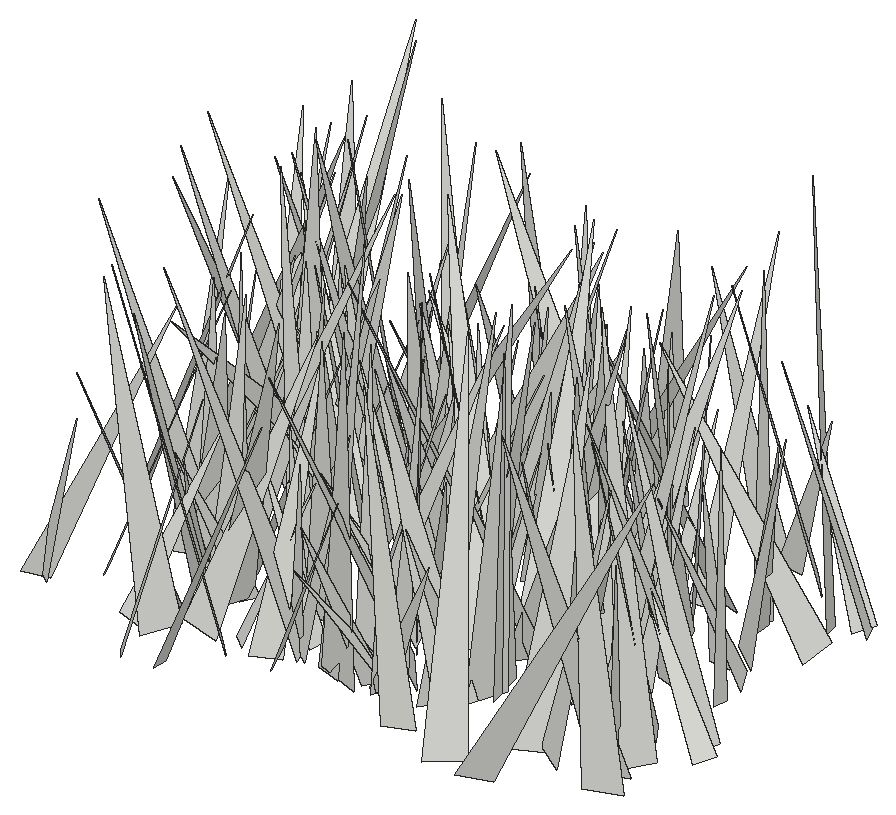
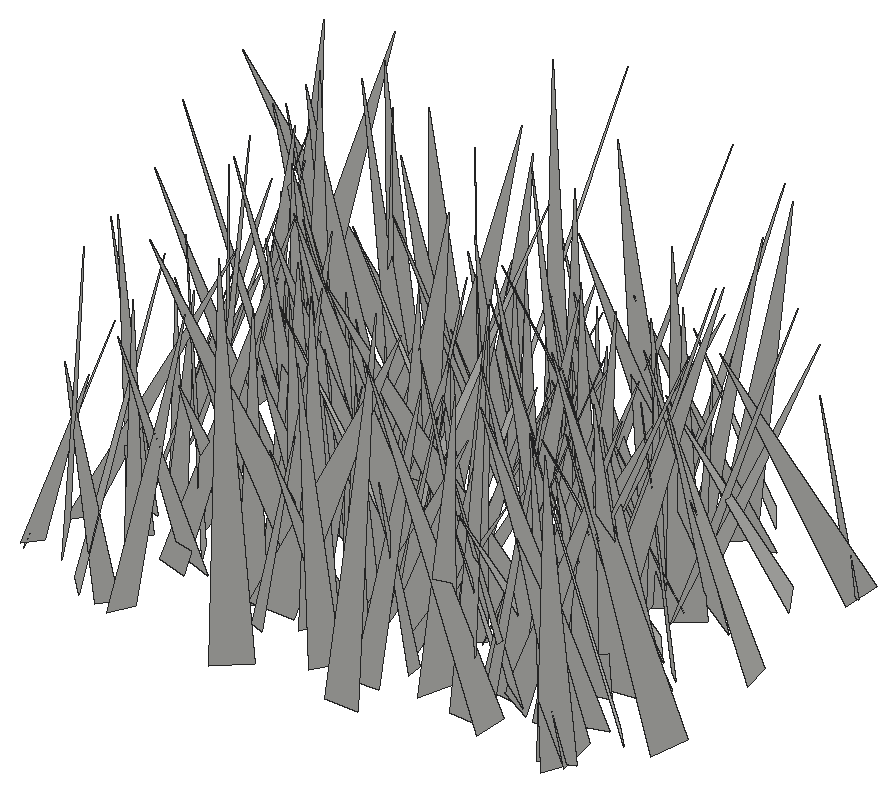
# SketchUp Ruby script. Lengths in inches.
U = 1.inch
M = Sketchup.active_model
def pt(a) = Geom::Point3d.new(a.map { |v| v * U })
def face(e, loops, mat)
  f = e.add_face(loops[0].map { |a| pt(a) })
  loops[1..].each { |l| e.add_face(l.map { |a| pt(a) }).erase! }
  f.material = f.back_material = mat if mat
  f
end
# faces: each face lists its corners as indices into pts; further lists are holes
def faces(e, pts, list, mat = nil) = list.each { |f| face(e, (f[0].is_a?(Array) ? f : [f]).map { |l| l.map { |i| pts[i] } }, mat) }
# xy, xz, yz: faces in a plane at the given z, y or x. An outline is a flat list of corners, or four numbers for a rectangle; further outlines are holes
def ring(l) = l.size == 4 ? [[l[0], l[1]], [l[2], l[1]], [l[2], l[3]], [l[0], l[3]]] : l.each_slice(2).to_a
def flat(e, list, mat, &to3) = list.each { |f| face(e, (f[0].is_a?(Array) ? f : [f]).map { |l| ring(l).map { |u, v| to3.(u, v) } }, mat) }
def xy(e, z, list, mat = nil) = flat(e, list, mat) { |x, y| [x, y, z] }
def xz(e, y, list, mat = nil) = flat(e, list, mat) { |x, z| [x, y, z] }
def yz(e, x, list, mat = nil) = flat(e, list, mat) { |y, z| [x, y, z] }
def lines(e, pts, list) = list.each { |a, b| e.add_line(pt(pts[a]), pt(pts[b])) }
# prism: a flat outline (further loops are holes) pulled along v
def prism(e, loops, v, mat = nil)
  f = face(e, loops, mat); d = Geom::Vector3d.new(v.map { |x| x * U })
  f.pushpull(f.normal.samedirection?(d) ? d.length : -d.length)
end
def box(e, o, s, mat = nil) = prism(e, [[o, [o[0] + s[0], o[1], o[2]], [o[0] + s[0], o[1] + s[1], o[2]], [o[0], o[1] + s[1], o[2]]]], [0, 0, s[2]], mat)
def at(x, y, z, deg = 0) = Geom::Transformation.translation(pt([x, y, z])) * Geom::Transformation.rotation(ORIGIN, Z_AXIS, deg.degrees)
def axes(o, x, y, z) = Geom::Transformation.new([*x, 0, *y, 0, *z, 0, *pt(o).to_a, 1])
def part(name) = M.definitions.add(name)
# library, detail: a bought-in or finely detailed component or shape, given as its bounding box
def library(name, o, s) = part(name).tap { |d| box(d.entities, o, s) }
def detail(e, o, s) = box(e.add_group.entities, o, s)
def put(e, d, t, mat = nil) = e.add_instance(d, t).tap { |i| i.material = mat if mat }
def group(e, t, mat = nil) = e.add_group.tap { |g| g.transformation = t; g.material = mat if mat }.entities
root = M.entities
c1 = part("fur_instance\#9")
p = [[0.8125,0,1.79],[0.67,-0.02,1.48],[0,-0.11,0],[0,0.11,0]]
faces(c1.entities,p,[[0,1,2,3]])
put(root,c1,axes([93.47,217.7,-27.1],[-5.98098,3.27291,2.42019],[3.72115,6.13978,0.89298],[1.64993,-1.98304,6.75918]))
put(root,c1,axes([94.98,215.74,-27.1],[4.77629,1.47467,0.59608],[1.29577,-4.70156,1.24867],[-0.92247,1.03128,4.84029]))
put(root,c1,axes([93.41,215.47,-27.1],[3.76197,3.17485,0.58422],[2.97684,-3.75885,1.25811],[-1.24876,0.60394,4.75913]))
put(root,c1,axes([102.43,220.92,-27.1],[-6.0329,-5.73941,0.68236],[-5.34499,5.91535,2.49841],[2.19943,-1.36753,7.94322]))
put(root,c1,axes([97.98,218.64,-27.1],[5.19096,1.17327,0.15724],[1.14991,-4.82989,-1.92283],[0.28108,-1.90867,4.96239]))
put(root,c1,axes([95.97,218.12,-27.1],[-5.67662,-5.13617,1.32256],[-5.29359,5.60645,-0.94818],[0.32758,1.59402,7.59639]))
put(root,c1,axes([108.84,216.25,-27.1],[6.56364,-3.25708,1.01889],[-3.38805,-5.95385,2.79299],[0.40967,2.94467,6.77415]))
put(root,c1,axes([100.55,218.85,-27.1],[-1.23371,-7.71978,2.49826],[-7.92295,1.69122,1.31342],[1.75022,2.21429,7.70662]))
put(root,c1,axes([104.48,217.4,-27.1],[-1.23354,6.12021,2.2306],[6.48252,0.93032,1.03231],[-0.63996,-2.37312,6.15735]))
put(root,c1,axes([102.16,219.85,-27.1],[-3.24466,-1.65637,0.06319],[-1.44148,2.88818,1.68993],[0.81834,-1.47993,3.2273]))
put(root,c1,axes([101.77,219.4,-27.1],[1.92833,-3.54748,0.58332],[-3.33012,-2.01195,-1.22706],[-1.35468,-0.10385,3.84674]))
put(root,c1,axes([112.54,219.42,-27.1],[0.14854,-7.36709,1.66817],[-7.40985,-0.46607,-1.39849],[-1.46661,1.60862,7.23466]))
put(root,c1,axes([87.66,218.23,-27.1],[2.1321,2.91958,1.28602],[3.18698,-1.87905,-1.01782],[0.14466,-1.63367,3.46899]))
put(root,c1,axes([102.47,218.9,-27.1],[1.15805,-3.96128,0.43832],[-3.70743,-0.90324,1.63219],[1.46246,0.84697,3.79062]))
put(root,c1,axes([113.02,218.3,-27.1],[1.15068,-6.84996,3.27998],[-7.48842,-1.57649,-0.66528],[-1.26644,3.09791,6.914]))
put(root,c1,axes([98.26,219.91,-27.1],[-7.76303,-2.55675,1.09489],[-2.43873,7.81802,0.96517],[1.33728,-0.58482,8.11604]))
put(root,c1,axes([93.29,219.18,-27.1],[-3.10953,-4.00727,0.37973],[-3.98696,3.00024,-0.98706],[-0.55366,0.90108,4.97525]))
put(root,c1,axes([102.33,219.09,-27.1],[3.31226,-1.52366,0.97308],[-1.49474,-3.45052,-0.31491],[-1.01694,0.10903,3.63228]))
put(root,c1,axes([107.26,216.53,-27.1],[5.53383,-2.65462,5.00816],[-4.23304,-6.59023,1.18414],[-3.76962,3.5034,6.0223]))
put(root,c1,axes([92.13,217.6,-27.1],[0.26684,4.21608,0.5662],[4.07293,-0.08948,-1.25314],[1.22767,-0.6195,4.03438]))
put(root,c1,axes([105.17,219.86,-27.1],[4.68158,-4.31782,3.21331],[-4.18207,-5.59908,-1.43065],[-3.3881,0.94493,6.20597]))
put(root,c1,axes([104.95,220.79,-27.1],[4.08531,-1.79648,1.28746],[-1.24322,-4.1049,-1.78292],[-1.82737,-1.22355,4.09124]))
put(root,c1,axes([93.17,220.53,-27.1],[-2.27159,-6.08211,1.19958],[-6.16809,2.34544,0.21162],[0.62109,1.04786,6.48903]))
put(root,c1,axes([110.01,219.02,-27.1],[3.01267,4.99828,1.819],[5.31773,-2.78497,-1.15474],[0.11548,-2.15148,5.72063]))
put(root,c1,axes([94.23,220.75,-27.1],[7.12513,-3.29011,0.44393],[-3.26274,-7.13377,-0.50321],[-0.6135,-0.27186,7.83192]))
put(root,c1,axes([98,219.7,-27.1],[-1.12295,-3.74744,1.45837],[-3.89173,1.39395,0.58526],[1.01223,1.20198,3.86805]))
put(root,c1,axes([94.55,218.55,-27.1],[0.24671,6.36494,1.6516],[6.30189,0.24313,-1.87833],[1.87786,-1.65213,6.08648]))
put(root,c1,axes([96.19,218.75,-27.1],[2.19151,2.85606,0.09461],[2.85445,-2.18225,-0.24214],[0.13471,-0.22234,3.59182]))
put(root,c1,axes([98.43,219.36,-27.1],[2.5994,3.80823,1.24151],[3.99906,-2.55122,-0.54734],[-0.2268,-1.33772,4.57819]))
put(root,c1,axes([112.28,219.92,-27.1],[3.8396,0.83392,1.68617],[0.96833,-4.16197,-0.14664],[-1.61273,-0.51356,3.92638]))
put(root,c1,axes([87.5,218.04,-27.1],[5.30796,-1.91017,1.71118],[-2.50762,-4.68997,2.54311],[-0.53734,3.01775,5.03546]))
put(root,c1,axes([91.82,221.96,-27.1],[4.12034,-0.14152,0.59374],[0.17297,-3.61498,-2.06197],[-0.58535,-2.06437,3.57009]))
put(root,c1,axes([94.5625,221.38,-27.1],[1.61464,-3.26071,0.69447],[-2.99454,-1.75765,-1.29032],[-1.46534,-0.00102,3.40211]))
put(root,c1,axes([97.64,218.44,-27.1],[-4.32625,3.6169,1.13686],[3.35652,4.45591,-1.40339],[1.76301,0.39209,5.46158]))
put(root,c1,axes([98.51,220.31,-27.1],[-3.79909,0.62191,0.11225],[0.62576,3.79759,0.13861],[0.08831,-0.15497,3.84716]))
put(root,c1,axes([103.35,218.62,-27.1],[-6.05732,0.47074,1.68041],[-0.07648,5.99257,-1.95441],[1.74342,1.89841,5.75265]))
put(root,c1,axes([109.24,219.08,-27.1],[-4.71435,5.59524,2.23508],[5.56124,5.13291,-1.11952],[2.31839,-0.93486,7.23039]))
put(root,c1,axes([97.51,221.81,-27.1],[0.93072,-6.54849,1.55591],[-6.7031,-0.75944,0.81335],[0.60996,1.64631,6.5641]))
put(root,c1,axes([100.09,218.93,-27.1],[3.45024,7.01244,2.07893],[6.95776,-3.8555,1.45774],[-2.25516,-1.1667,7.67811]))
put(root,c1,axes([97.52,220.7,-27.1],[0.08392,3.77547,1.67654],[4.10941,-0.2474,0.35143],[-0.42151,-1.66031,3.76001]))
put(root,c1,axes([105.5625,221.02,-27.1],[7.52534,-2.11015,2.94691],[-2.32099,-8.02168,0.183],[-2.78389,0.98374,7.81345]))
put(root,c1,axes([104.37,219.53,-27.1],[-6.74927,1.80081,2.69667],[1.18797,7.16726,-1.81295],[3.01723,1.2063,6.74602]))
put(root,c1,axes([105.72,221.88,-27.1],[-6.42267,-1.42598,3.31634],[-1.29179,7.22813,0.60623],[3.37087,0.05298,6.55107]))
put(root,c1,axes([91.19,223.32,-27.1],[3.73638,-5.69312,0.32255],[-5.69521,-3.70663,0.54933],[0.28337,0.57053,6.78752]))
put(root,c1,axes([101.1,222.87,-27.1],[-3.84083,-1.16764,0.10273],[-1.10793,3.73134,0.98769],[0.38264,-0.91633,3.89099]))
put(root,c1,axes([104.73,221.85,-27.1],[7.78387,0.2727,2.09642],[0.3333,-8.05673,-0.18953],[-2.08764,-0.26953,7.78634]))
put(root,c1,axes([100.16,220.98,-27.1],[1.00537,5.49165,1.69021],[5.63183,-1.28199,0.81538],[-1.13911,-1.49133,5.52306]))
put(root,c1,axes([101.02,222.72,-27.1],[5.50119,4.10651,2.99111],[4.73487,-5.74232,-0.82461],[-1.84151,-2.49711,6.81516]))
put(root,c1,axes([89.3,219.79,-27.1],[4.7893,3.01055,0.30481],[2.77693,-4.59952,1.79634],[-1.20208,1.36921,5.36414]))
put(root,c1,axes([93.03,221.77,-27.1],[4.88657,-1.90502,2.44295],[-2.30886,-5.28158,0.49977],[-2.06549,1.39696,5.22091]))
put(root,c1,axes([111.91,222.78,-27.1],[-4.7875,-3.33897,1.34753],[-3.4677,4.87923,-0.23006],[0.96934,0.96392,5.83232]))
put(root,c1,axes([91.79,222.45,-27.1],[0.33576,5.45677,2.6197],[6.05197,-0.25349,-0.24764],[0.11336,-2.62894,5.46148]))
put(root,c1,axes([91.74,222.99,-27.1],[-7.05109,-1.52018,0.70264],[-1.52291,7.08527,0.04653],[0.69669,0.10238,7.21295]))
put(root,c1,axes([99.61,224.15,-27.1],[-4.59032,-0.23962,0.17171],[-0.16134,4.28449,1.66587],[0.24672,-1.65642,4.28408]))
put(root,c1,axes([114.41,222.35,-27.1],[-3.16167,2.60611,0.16715],[2.5519,3.02748,1.0668],[-0.55458,-0.92652,3.956]))
put(root,c1,axes([113.07,223.96,-27.1],[-6.09562,-2.74651,0.83103],[-2.67616,6.14538,0.68045],[1.03541,-0.28555,6.65108]))
put(root,c1,axes([112.82,220.56,-27.1],[-8.1921,1.36867,0.61461],[1.20152,8.02801,-1.8625],[0.89853,1.74336,8.09413]))
put(root,c1,axes([105.68,224.04,-27.1],[-0.21744,-4.53269,0.61909],[-4.46943,0.07824,-0.99696],[-0.9761,0.65149,4.42703]))
put(root,c1,axes([92.64,223.16,-27.1],[0.05129,-4.93553,2.34933],[-4.99892,0.90807,2.01684],[2.21125,2.16734,4.50493]))
put(root,c1,axes([99.3125,221.97,-27.1],[3.76049,3.04894,0.61025],[2.98388,-3.80785,0.6375],[-0.87456,0.11813,4.79905]))
put(root,c1,axes([99.18,222.4,-27.1],[3.55811,5.92159,0.8478],[5.93377,-3.36884,-1.37307],[0.75783,-1.4247,6.77052]))
put(root,c1,axes([105.36,226.57,-27.1],[1.43301,-8.2393,0.15598],[-8.02359,-1.35888,1.93375],[1.87948,0.48092,8.13635]))
put(root,c1,axes([113.97,222.97,-27.1],[-6.67851,0.63047,0.27765],[0.60623,6.66388,-0.54986],[0.32721,0.52189,6.68563]))
put(root,c1,axes([92.96,222.83,-27.1],[-5.66532,-0.50223,1.85308],[-0.88322,5.80808,-1.12609],[1.70472,1.34012,5.57494]))
put(root,c1,axes([93.61,222.64,-27.1],[4.63443,1.21877,0.59299],[1.09033,-4.6073,0.94811],[-0.80513,0.77609,4.69728]))
put(root,c1,axes([104.89,224.11,-27.1],[7.07738,-3.29601,0.99897],[-3.4049,-7.03943,0.89669],[-0.51794,1.23844,7.75557]))
put(root,c1,axes([100.48,223.4375,-27.1],[5.45999,3.37552,0.2587],[3.37248,-5.38033,-0.97518],[0.29572,-0.96459,6.34466]))
put(root,c1,axes([106.65,225.87,-27.1],[1.50872,-5.62418,0.24688],[-5.60162,-1.47433,0.64555],[0.56049,0.40439,5.78713]))
put(root,c1,axes([99.46,225.96,-27.1],[-0.15941,-4.26775,0.08772],[-3.87813,0.18147,1.78158],[1.78369,0.01316,3.88138]))
put(root,c1,axes([100.71,226.11,-27.1],[1.73584,-5.70606,0.92261],[-5.63591,-1.88469,-1.0526],[-1.28332,0.55882,5.87063]))
put(root,c1,axes([110.05,222.13,-27.1],[3.85814,7.37241,1.12129],[7.37277,-3.96052,0.67189],[-1.11889,-0.67587,8.29374]))
put(root,c1,axes([101.55,227.35,-27.1],[-5.30348,-5.59312,0.1785],[-5.55783,5.29332,0.73008],[0.65218,-0.37354,7.67313]))
put(root,c1,axes([95.92,222.74,-27.1],[-7.72963,0.57294,0.92033],[0.30078,7.49944,-2.14251],[1.04153,2.08628,7.44883]))
put(root,c1,axes([99.85,224.42,-27.1],[-4.67921,0.76999,0.1435],[0.76372,4.67821,-0.1991],[0.17382,0.17327,4.73796]))
put(root,c1,axes([108.08,223.07,-27.1],[6.4621,3.38539,1.99868],[3.00841,-6.73382,1.67909],[-2.53082,0.63956,7.09931]))
put(root,c1,axes([91.97,222.72,-27.1],[4.66085,6.54813,0.11631],[6.5407,-4.64683,-0.4912],[0.3329,-0.37945,8.02249]))
put(root,c1,axes([93.57,229.97,-27.1],[5.32765,-5.22538,0.29084],[-4.03169,-4.36253,-4.52625],[-3.33686,-3.07194,5.93309]))
put(root,c1,axes([90.4375,222.5,-27.1],[2.16067,6.65454,0.44246],[6.23565,-2.18071,2.34697],[-2.36543,0.32979,6.59114]))
put(root,c1,axes([103.35,223.97,-27.1],[-5.00695,6.61488,0.9269],[6.67749,4.92855,0.89773],[-0.16413,-1.27989,8.24744]))
put(root,c1,axes([86.73,224.94,-27.1],[6.39935,1.66924,0.57136],[1.67346,-6.42366,0.02366],[-0.55885,-0.12123,6.61343]))
put(root,c1,axes([94.04,227.03,-27.1],[1.95757,-4.55386,0.31612],[-4.56359,-1.94437,0.25034],[0.10577,0.38911,4.95045]))
put(root,c1,axes([102.51,224.93,-27.1],[-0.54447,5.56352,1.73211],[5.79599,0.33809,0.73596],[-0.59958,-1.78391,5.54144]))
put(root,c1,axes([109.8125,225.92,-27.1],[-2.15143,-4.58063,1.63472],[-4.86135,2.07952,-0.57094],[0.14745,1.72526,5.02841]))
put(root,c1,axes([104.61,226.17,-27.1],[-1.9321,-3.03286,0.9193],[-3.13143,1.99261,-0.00754],[0.48737,0.77951,3.596]))
put(root,c1,axes([101.43,226.6,-27.1],[3.99613,2.0991,0.80323],[2.24013,-3.58697,-1.77087],[0.18236,-1.93595,4.15203]))
put(root,c1,axes([109.92,226.05,-27.1],[4.37424,4.04681,2.79179],[4.54542,-4.75288,-0.23239],[-1.87347,-2.08284,5.95454]))
put(root,c1,axes([92.67,227.01,-27.1],[-7.47727,-2.4998,1.10622],[-2.44373,7.5564,0.55783],[1.22512,-0.18436,7.86431]))
put(root,c1,axes([103.01,224.3,-27.1],[-1.19348,5.65379,0.3473],[5.3271,0.99964,2.033],[-1.92561,-0.73875,5.40894]))
put(root,c1,axes([111.91,227.6875,-27.1],[-4.09527,-2.1175,0.66115],[-1.87882,4.04889,1.32991],[1.17939,-0.90267,4.41434]))
put(root,c1,axes([93.14,226.29,-27.1],[5.23095,-0.44242,1.6949],[-0.413,-5.49862,-0.16069],[-1.70231,-0.02548,5.24716]))
put(root,c1,axes([90.93,229.12,-27.1],[-1.44964,-7.72306,0.36058],[-7.72764,1.4358,-0.315],[-0.24346,0.41228,7.85162]))
put(root,c1,axes([89.07,226.7,-27.1],[3.62429,3.41254,1.71474],[3.78655,-3.51895,-1.00013],[-0.49783,-1.92166,4.87654]))
put(root,c1,axes([105.39,228.53,-27.1],[5.27759,-3.33069,0.22963],[-3.2336,-5.20637,-1.19863],[-0.83073,-0.89406,6.12452]))
put(root,c1,axes([96.05,226.33,-27.1],[-3.65286,-4.07637,1.60167],[-4.37583,3.48496,-1.11027],[0.18514,1.94004,5.3598]))
put(root,c1,axes([107.84,224.27,-27.1],[0.68594,6.83231,0.78357],[6.74689,-0.82108,1.2531],[-1.33188,-0.64057,6.75135]))
put(root,c1,axes([109.4,225.08,-27.1],[1.25627,4.75609,0.70963],[4.78282,-1.31187,0.32531],[-0.49861,-0.60066,4.90844]))
put(root,c1,axes([104.28,227.19,-27.1],[-2.25784,-3.06403,1.232],[-3.11024,2.47464,0.4545],[1.1102,0.70132,3.77883]))
put(root,c1,axes([100.89,227.49,-27.1],[3.77255,3.78798,3.73229],[4.48771,-4.72284,0.25719],[-2.85294,-2.4201,5.33992]))
put(root,c1,axes([105.02,224.56,-27.1],[-3.53884,7.24303,1.02774],[7.25201,3.62348,-0.56563],[0.96238,-0.67082,8.04145]))
put(root,c1,axes([97.62,227.125,-27.1],[2.40925,-3.29701,1.00546],[-3.44676,-2.29271,0.74099],[0.03277,1.24857,4.01568]))
put(root,c1,axes([112.3,225.875,-27.1],[-4.48133,-0.60292,1.35721],[-0.97091,4.45413,-1.22715],[1.12377,1.44397,4.35201]))
put(root,c1,axes([104.21,228.64,-27.1],[6.83248,-2.68093,1.04491],[-2.55055,-6.88917,-0.99801],[-1.33189,-0.56029,7.27146]))
put(root,c1,axes([100.55,227.27,-27.1],[-3.18222,-1.83698,0.96818],[-1.93012,3.2701,-0.13938],[0.76583,0.60852,3.67173]))
put(root,c1,axes([94.68,224.61,-27.1],[4.61652,6.22378,1.13894],[6.03614,-4.75491,1.51682],[-1.89675,0.0163,7.59914]))
put(root,c1,axes([108.72,228.5,-27.1],[-6.30807,-3.21691,2.7037],[-2.95993,6.86307,1.25992],[2.98285,0.00727,6.96799]))
put(root,c1,axes([101.82,228.58,-27.1],[2.32363,-4.81619,0.47979],[-4.81966,-2.25368,0.71896],[0.44354,0.74187,5.29887]))
put(root,c1,axes([90.77,225.29,-27.1],[3.00596,2.69315,0.13963],[2.45938,-2.82346,1.51258],[-1.10635,1.04086,3.74179]))
put(root,c1,axes([110.53,228.07,-27.1],[0.0054,-4.02258,1.09842],[-4.16704,0.03516,0.14925],[0.15324,1.09787,4.01982]))
put(root,c1,axes([103.375,227.09,-27.1],[3.80415,1.70942,1.42934],[1.7089,-4.05302,0.29902],[-1.42996,-0.29602,4.15984]))
put(root,c1,axes([106.6,226.08,-27.1],[-4.20959,5.12778,0.85898],[5.1677,4.24809,-0.03415],[0.57165,-0.64206,6.63427]))
put(root,c1,axes([105.72,228.33,-27.1],[0.0044,-6.27087,2.13822],[-6.5778,-0.25997,-0.7489],[-0.79272,2.12236,6.226]))
put(root,c1,axes([99.6875,228.45,-27.1],[2.95462,-6.48005,1.02046],[-5.97059,-2.19282,3.36242],[2.71745,2.2277,6.27814]))
put(root,c1,axes([101.51,226.65,-27.1],[2.79902,6.82497,1.56007],[7.00009,-2.70115,-0.74237],[0.11309,-1.72399,7.33919]))
put(root,c1,axes([106.88,226.2,-27.1],[1.72672,7.47142,1.23195],[7.48463,-1.49226,-1.44043],[1.14896,-1.50745,7.53186]))
put(root,c1,axes([96.29,229.27,-27.1],[4.8862,-3.80667,1.31151],[-3.74132,-5.05482,-0.73291],[-1.48774,0.20937,6.1505]))
put(root,c1,axes([105.53,226.4375,-27.1],[-3.3116,2.69695,0.72945],[2.42136,3.33487,-1.33716],[1.39378,0.61437,4.05614]))
put(root,c1,axes([91.51,228.21,-27.1],[2.46407,-3.91283,1.91735],[-4.25122,-2.64198,0.07181],[-0.95581,1.66367,4.6235]))
put(root,c1,axes([93.38,228.4,-27.1],[-7.85705,-0.88135,0.16267],[-0.88597,7.85465,-0.23661],[0.1352,0.25331,7.90278]))
put(root,c1,axes([88.35,227.79,-27.1],[3.49532,2.40186,0.16337],[2.40303,-3.46356,-0.49202],[0.14512,-0.49771,4.21237]))
put(root,c1,axes([92.17,228.77,-27.1],[1.0853,-7.02468,2.48253],[-7.23303,-0.3918,2.05344],[1.78669,2.68091,6.80495]))
put(root,c1,axes([110.92,228.98,-27.1],[-1.89095,-4.65132,2.366],[-4.60338,2.67208,1.57395],[2.45798,1.42605,4.76793]))
put(root,c1,axes([96.24,228.15,-27.1],[-6.99068,-2.50094,0.47101],[-2.54423,6.83653,-1.46112],[-0.05835,1.53405,7.27938]))
put(root,c1,axes([87.7,229.24,-27.1],[1.22983,-5.08709,1.30795],[-5.046,-0.77126,1.74491],[1.45845,1.62123,4.93419]))
put(root,c1,axes([95.33,227.19,-27.1],[7.21653,-2.33327,0.39687],[-2.31249,-6.67999,2.77668],[0.50399,2.75925,7.05779]))
put(root,c1,axes([90.52,229.59,-27.1],[1.05516,-7.50337,2.43147],[-7.87164,-0.84629,0.8044],[0.49989,2.51181,7.53438]))
put(root,c1,axes([90.88,225.31,-27.1],[4.07419,5.57288,0.07978],[5.18286,-3.82462,2.48447],[-2.04971,1.40628,6.44076]))
put(root,c1,axes([94.53,227.4375,-27.1],[-3.04335,5.85133,0.32291],[5.70958,2.87864,1.64877],[-1.32023,-1.03909,6.38604]))
put(root,c1,axes([110.125,230.6,-27.1],[5.73315,-1.08828,0.33068],[-0.98004,-5.58896,-1.40205],[-0.57725,-1.3198,5.66459]))
put(root,c1,axes([107.92,231.625,-27.1],[-1.99035,-6.59495,0.1128],[-6.59501,1.99173,0.07994],[0.10913,0.08488,6.88828]))
put(root,c1,axes([97.71,229.28,-27.1],[4.40599,-6.63506,1.39046],[-6.52465,-3.70025,3.01783],[1.84021,2.76664,7.37085]))
put(root,c1,axes([92.23,227.47,-27.1],[-0.89857,4.82904,0.37817],[4.8418,0.88433,0.21213],[-0.14006,-0.41036,4.90735]))
put(root,c1,axes([93.55,229.64,-27.1],[3.00214,-3.52749,1.91618],[-3.65397,-3.39209,-0.51969],[-1.66236,1.08552,4.60282]))
put(root,c1,axes([106.88,228.03,-27.1],[2.68485,5.08236,0.90598],[5.15716,-2.6868,-0.21076],[-0.23424,-0.9002,5.74408]))
put(root,c1,axes([87.57,229.16,-27.1],[5.01329,4.55618,1.17415],[4.70331,-4.80639,-1.43108],[0.12753,-1.84671,6.62147]))
put(root,c1,axes([100.75,226.8,-27.1],[4.99959,5.18328,0.38062],[5.01525,-4.9501,1.53324],[-1.36326,0.79826,7.03643]))
put(root,c1,axes([108.39,227.45,-27.1],[-3.90191,2.21296,0.38649],[1.88444,3.64598,-1.85127],[1.22289,1.44261,4.08594]))
put(root,c1,axes([100.03,230.125,-27.1],[-1.04898,-5.12431,2.12616],[-5.35306,1.50327,0.98203],[1.45734,1.83333,5.13756]))
put(root,c1,axes([112.7,230.87,-27.1],[-6.59727,0.97904,0.29915],[1.02311,6.37288,1.70633],[0.03533,-1.73199,6.44755]))
put(root,c1,axes([103.26,230,-27.1],[2.23095,-4.80055,1.901],[-5.14348,-2.24733,0.36107],[-0.45138,1.8816,5.28129]))
put(root,c1,axes([93.06,231.61,-27.1],[-0.40917,-7.70862,1.45343],[-7.84037,0.35495,-0.32469],[-0.25296,1.46762,7.71264]))
put(root,c1,axes([107.66,230.13,-27.1],[5.0794,2.90769,2.21904],[3.29641,-5.28463,-0.62087],[-1.58507,-1.67247,5.81975]))
put(root,c1,axes([103.52,228.36,-27.1],[-5.59441,-0.96055,0.72122],[-1.15543,5.24244,-1.98041],[0.32833,2.08191,5.31959]))
put(root,c1,axes([100.04,229.82,-27.1],[-3.98181,3.20015,0.16473],[3.12043,3.81261,1.36007],[-0.7287,-1.16015,4.92402]))
put(root,c1,axes([99.5625,229.46,-27.1],[-5.02924,-0.94611,0.83871],[-1.10156,4.96734,-1.00192],[0.62059,1.14984,5.01842]))
put(root,c1,axes([89.83,228.86,-27.1],[-1.61925,6.67608,1.38838],[6.8184,1.60284,0.24489],[0.08425,-1.4073,6.86528]))
put(root,c1,axes([89.64,228,-27.1],[2.76869,6.15296,0.77217],[6.00563,-2.8712,1.34513],[-1.54517,-0.13446,6.61174]))
put(root,c1,axes([104.3,229.97,-27.1],[1.80379,6.11401,2.80003],[6.29213,-2.55743,1.53087],[-2.37284,-2.13386,6.18799]))
put(root,c1,axes([97.13,227.83,-27.1],[3.53249,6.50702,1.2231],[6.07163,-3.73652,2.34297],[-2.64057,0.11331,7.02355]))
put(root,c1,axes([85.97,230.83,-27.1],[7.43524,-1.67911,0.29476],[-1.69435,-7.42416,0.44731],[-0.18841,0.50147,7.60934]))
put(root,c1,axes([90.39,232.38,-27.1],[-0.97227,-5.54065,0.71566],[-5.53732,1.05209,0.62249],[0.741,0.5921,5.59077]))
put(root,c1,axes([99.91,231.23,-27.1],[4.11916,-1.93041,1.42636],[-1.9279,-4.34864,-0.31782],[-1.42975,0.30221,4.53795]))
put(root,c1,axes([96.21,231.24,-27.1],[1.60844,-3.68609,1.55705],[-3.78668,-1.94455,-0.69177],[-1.29334,1.10916,3.96179]))
put(root,c1,axes([97.53,231.12,-27.1],[-2.45268,-3.25533,0.28731],[-3.08329,2.18606,-1.55237],[-1.08306,1.14864,3.76868]))
put(root,c1,axes([103.95,231.99,-27.1],[4.8037,-2.51399,0.9877],[-2.43404,-4.90267,-0.64073],[-1.17095,-0.12226,5.38379]))
put(root,c1,axes([92.3125,229.05,-27.1],[3.84867,2.11329,0.22175],[1.92609,-3.66331,1.48248],[-0.8974,1.20066,4.13285]))
put(root,c1,axes([92.2,231.79,-27.1],[-2.37076,-5.83706,1.32394],[-5.9146,2.06646,-1.48049],[-0.91737,1.76156,6.12372]))
put(root,c1,axes([101.71,230.44,-27.1],[7.5928,-1.32868,0.07278],[-1.31152,-7.40102,1.71058],[0.22497,1.69728,7.51598]))
put(root,c1,axes([93.06,232.18,-27.1],[-4.49464,-4.79472,1.8462],[-5.03521,4.59856,-0.3156],[1.02201,1.56958,6.56442]))
put(root,c1,axes([105.22,231.42,-27.1],[4.42317,-1.03576,2.17466],[-1.28949,-4.85884,0.30856],[-2.03449,0.82776,4.53233]))
put(root,c1,axes([93.09,233.73,-27.1],[-1.97553,-6.78705,1.45707],[-6.65434,2.28292,1.61176],[1.97656,0.90224,6.88251]))
put(root,c1,axes([101.17,231.7,-27.1],[-5.47966,3.19166,2.7493],[3.39794,6.01513,-0.2105],[2.48986,-1.18473,6.33791]))
put(root,c1,axes([94.47,229.89,-27.1],[2.91558,3.30379,0.88214],[2.68077,-2.92801,2.10571],[-2.12289,0.83996,3.8706]))
put(root,c1,axes([97.2,234.02,-27.1],[-0.08674,-5.50292,0.32115],[-5.49794,0.10952,0.39174],[0.3974,0.31411,5.48965]))
put(root,c1,axes([102.82,233.17,-27.1],[-1.51621,-3.26203,0.55212],[-3.23761,1.58793,0.49084],[0.68086,0.28668,3.56354]))
put(root,c1,axes([96.5,232.13,-27.1],[3.55375,0.65284,0.74182],[0.70307,-3.6162,-0.18565],[-0.69441,-0.32026,3.60844]))
put(root,c1,axes([92.18,231.6875,-27.1],[2.56604,4.25646,1.10853],[4.39439,-2.42581,-0.85772],[0.18887,-1.38883,4.89555]))
put(root,c1,axes([103.17,231.89,-27.1],[-4.31341,6.46311,1.11663],[6.32564,3.74609,2.75266],[-1.73345,-2.41229,7.26637]))
put(root,c1,axes([89.99,232.32,-27.1],[-3.27969,0.65416,1.38528],[0.68941,3.5533,-0.04576],[1.36808,-0.22237,3.34398]))
put(root,c1,axes([101.04,231,-27.1],[4.03542,0.28371,1.50858],[-0.2798,-4.0361,1.5075],[-1.50932,1.50677,3.754]))
put(root,c1,axes([87.81,231.22,-27.1],[4.5925,4.65986,1.11021],[4.70947,-4.6734,0.13435],[-0.87619,-0.69491,6.5412]))
put(root,c1,axes([109.89,231.3,-27.1],[-6.28866,-0.36775,1.68536],[-0.82762,6.23312,-1.72806],[1.51351,1.8804,6.05775]))
put(root,c1,axes([113.26,233.17,-27.1],[-4.74174,-2.50609,0.51828],[-2.55748,4.67952,-0.77105],[0.09149,0.92453,5.30754]))
put(root,c1,axes([99.17,233.89,-27.1],[4.9839,-2.53795,0.76874],[-2.53211,-5.04073,-0.2255],[-0.78777,0.14572,5.58834]))
put(root,c1,axes([88.23,234.5625,-27.1],[6.05752,-0.57817,0.88939],[-0.39,-6.0087,-1.2499],[-0.9865,-1.17476,5.9553]))
put(root,c1,axes([109.7,234.78,-27.1],[-4.76298,-4.61729,1.21885],[-4.61962,4.89113,0.47635],[1.20999,0.49843,6.61653]))
put(root,c1,axes([112.93,233.25,-27.1],[-3.82314,1.91513,0.41484],[1.95484,3.79049,0.51675],[0.13566,-0.64863,4.24466]))
put(root,c1,axes([91.85,233.63,-27.1],[7.09843,0.26187,0.16049],[0.26265,-7.10014,-0.03187],[-0.15921,-0.03777,7.10319]))
put(root,c1,axes([94.99,232.74,-27.1],[-6.58758,2.43197,1.48528],[2.355,6.75255,-0.6115],[1.60454,0.07391,6.99549]))
put(root,c1,axes([107.4,231,-27.1],[1.20703,6.81999,0.05967],[6.70849,-1.19813,1.23829],[-1.22962,0.158,6.81439]))
put(root,c1,axes([89.15,231.48,-27.1],[-1.14842,8.02715,0.79991],[8.02073,1.22255,-0.75306],[0.86188,-0.68125,8.07384]))
put(root,c1,axes([101.82,235.83,-27.1],[5.04429,-5.44094,0.7168],[-5.46997,-5.06343,0.05905],[-0.44381,0.56596,7.41924]))
put(root,c1,axes([88.16,233.32,-27.1],[7.83085,1.1219,1.78667],[1.00117,-8.02181,0.64907],[-1.85702,0.40616,7.88414]))
put(root,c1,axes([108.1,235.05,-27.1],[1.41621,-4.16021,0.5332],[-4.01988,-1.18575,1.42542],[1.19673,0.94019,4.15706]))
put(root,c1,axes([96.97,235.67,-27.1],[-0.69172,-7.26259,1.83893],[-7.46362,0.82804,0.46276],[0.64909,1.78171,7.28077]))
put(root,c1,axes([107.41,235.1,-27.1],[-5.83631,0.9789,1.84731],[1.28037,6.00401,0.86359],[1.65271,-1.19453,5.85448]))
put(root,c1,axes([112.05,232.47,-27.1],[-7.32928,-2.99407,2.48715],[-3.76161,6.81126,-2.88543],[1.00033,3.67572,7.37273]))
put(root,c1,axes([88.4,234.17,-27.1],[-2.28357,5.70644,2.33564],[6.0895,2.47813,-0.10083],[0.96778,-2.12809,6.14557]))
